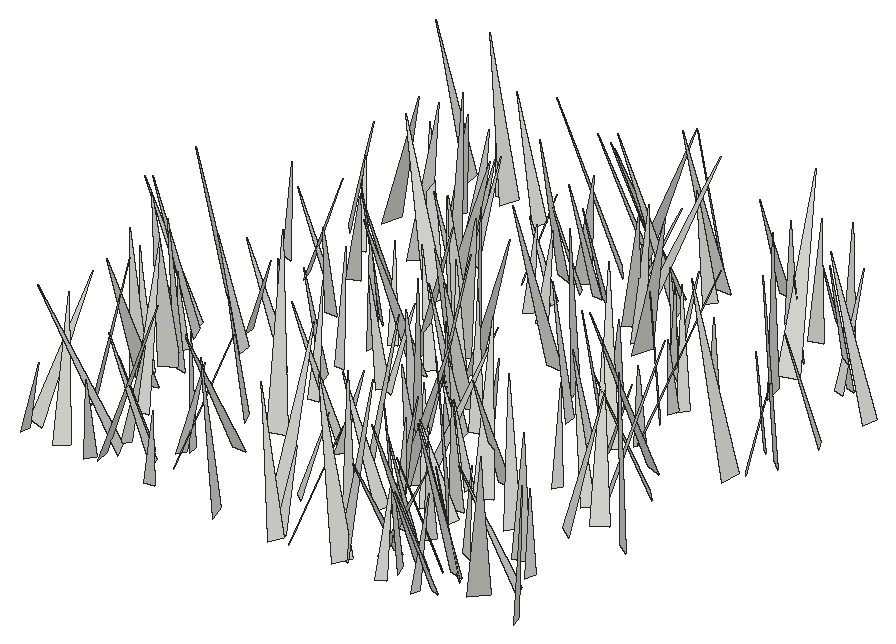
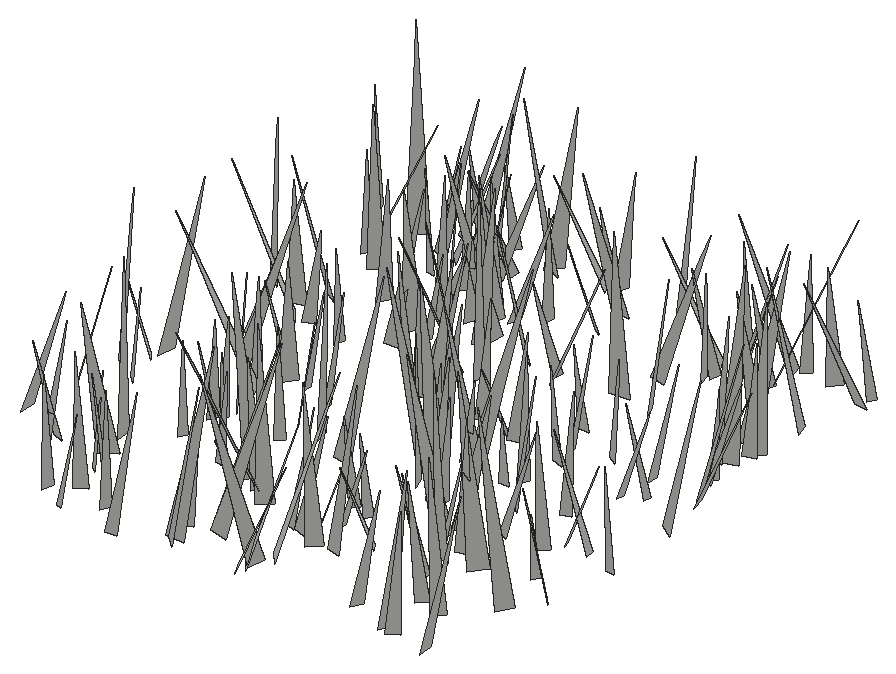
# SketchUp Ruby script. Lengths in inches.
U = 1.inch
M = Sketchup.active_model
def pt(a) = Geom::Point3d.new(a.map { |v| v * U })
def face(e, loops, mat)
  f = e.add_face(loops[0].map { |a| pt(a) })
  loops[1..].each { |l| e.add_face(l.map { |a| pt(a) }).erase! }
  f.material = f.back_material = mat if mat
  f
end
# faces: each face lists its corners as indices into pts; further lists are holes
def faces(e, pts, list, mat = nil) = list.each { |f| face(e, (f[0].is_a?(Array) ? f : [f]).map { |l| l.map { |i| pts[i] } }, mat) }
# xy, xz, yz: faces in a plane at the given z, y or x. An outline is a flat list of corners, or four numbers for a rectangle; further outlines are holes
def ring(l) = l.size == 4 ? [[l[0], l[1]], [l[2], l[1]], [l[2], l[3]], [l[0], l[3]]] : l.each_slice(2).to_a
def flat(e, list, mat, &to3) = list.each { |f| face(e, (f[0].is_a?(Array) ? f : [f]).map { |l| ring(l).map { |u, v| to3.(u, v) } }, mat) }
def xy(e, z, list, mat = nil) = flat(e, list, mat) { |x, y| [x, y, z] }
def xz(e, y, list, mat = nil) = flat(e, list, mat) { |x, z| [x, y, z] }
def yz(e, x, list, mat = nil) = flat(e, list, mat) { |y, z| [x, y, z] }
def lines(e, pts, list) = list.each { |a, b| e.add_line(pt(pts[a]), pt(pts[b])) }
# prism: a flat outline (further loops are holes) pulled along v
def prism(e, loops, v, mat = nil)
  f = face(e, loops, mat); d = Geom::Vector3d.new(v.map { |x| x * U })
  f.pushpull(f.normal.samedirection?(d) ? d.length : -d.length)
end
def box(e, o, s, mat = nil) = prism(e, [[o, [o[0] + s[0], o[1], o[2]], [o[0] + s[0], o[1] + s[1], o[2]], [o[0], o[1] + s[1], o[2]]]], [0, 0, s[2]], mat)
def at(x, y, z, deg = 0) = Geom::Transformation.translation(pt([x, y, z])) * Geom::Transformation.rotation(ORIGIN, Z_AXIS, deg.degrees)
def axes(o, x, y, z) = Geom::Transformation.new([*x, 0, *y, 0, *z, 0, *pt(o).to_a, 1])
def part(name) = M.definitions.add(name)
# library, detail: a bought-in or finely detailed component or shape, given as its bounding box
def library(name, o, s) = part(name).tap { |d| box(d.entities, o, s) }
def detail(e, o, s) = box(e.add_group.entities, o, s)
def put(e, d, t, mat = nil) = e.add_instance(d, t).tap { |i| i.material = mat if mat }
def group(e, t, mat = nil) = e.add_group.tap { |g| g.transformation = t; g.material = mat if mat }.entities
root = M.entities
c1 = part("fur_instance\#9")
p = [[0.8125,0,1.79],[0.67,-0.02,1.48],[0,-0.11,0],[0,0.11,0]]
faces(c1.entities,p,[[0,1,2,3]])
put(root,c1,axes([455.98,77.39,-21.66],[-6.00367,-1.40851,0.07652],[-1.40991,5.98159,-0.51624],[-0.04369,0.52005,6.14503]))
put(root,c1,axes([455.24,82.02,-21.66],[-3.32824,-5.52708,1.61735],[-5.74671,3.30884,-0.51825],[0.37393,1.65668,6.43096]))
put(root,c1,axes([454.55,89.52,-21.66],[-0.60793,-4.00143,1.69165],[-4.28266,0.83877,0.44495],[0.72934,1.58988,4.02282]))
put(root,c1,axes([456.5625,76.4,-21.66],[-6.28754,-2.52373,1.27093],[-2.51372,6.41179,0.29625],[1.29062,0.19325,6.76865]))
put(root,c1,axes([455.45,95.79,-21.66],[3.51843,3.11531,1.14482],[3.25687,-3.56198,-0.31656],[-0.63919,-1.00114,4.68874]))
put(root,c1,axes([457.41,74.3,-21.66],[-2.05359,-3.75931,0.63579],[-3.81243,2.01617,-0.39286],[-0.04503,0.74602,4.26559]))
put(root,c1,axes([455.75,58.35,-21.66],[1.29367,6.30142,0.29631],[6.29029,-1.26564,-0.54746],[0.47747,-0.39942,6.4095]))
put(root,c1,axes([457.89,107.22,-21.66],[-6.59248,-1.12335,1.64682],[-1.04061,6.79216,0.46743],[1.70031,-0.1986,6.67115]))
put(root,c1,axes([457.38,69.51,-21.66],[1.73924,-4.25815,2.51532],[-4.74882,-2.1825,-0.41111],[-1.38108,2.14207,4.58125]))
put(root,c1,axes([455.6875,57.11,-21.66],[3.70802,-0.97097,0.29213],[-0.94384,-3.70994,-0.3508],[-0.37053,-0.26665,3.81695]))
put(root,c1,axes([457.16,68.78,-21.66],[-4.56803,3.68378,2.77525],[4.20348,4.93276,0.37129],[1.89817,-2.05836,5.85656]))
put(root,c1,axes([457.33,73.82,-21.66],[2.92591,-1.89098,1.19539],[-1.88086,-3.14489,-0.37117],[-1.21125,0.31559,3.46396]))
put(root,c1,axes([458.28,93.65,-21.66],[-2.65941,2.49787,0.36396],[2.46932,2.68404,-0.37765],[0.52369,0.0288,3.62894]))
put(root,c1,axes([458.09,71.22,-21.66],[2.83404,-7.21043,2.36501],[-7.48804,-3.06648,-0.37599],[-1.22999,2.05469,7.73827]))
put(root,c1,axes([459.79,88.1,-21.66],[-3.92921,-1.09616,0.24918],[-1.11465,3.91653,-0.34741],[0.14562,0.40197,4.06442]))
put(root,c1,axes([456.86,63.92,-21.66],[6.14666,2.4589,1.36982],[2.59506,-6.2248,-0.47069],[-1.09008,-0.95377,6.60349]))
put(root,c1,axes([459,71.33,-21.66],[1.62899,5.48386,2.82302],[6.01922,-2.05055,0.50999],[-1.34582,-2.53344,5.69792]))
put(root,c1,axes([459.23,57.04,-21.66],[-4.06626,4.25963,1.22614],[4.27905,4.20638,-0.4224],[1.15655,-0.5867,5.87371]))
put(root,c1,axes([458.66,68.01,-21.66],[1.6119,-7.35068,0.1441],[-7.34568,-1.61634,-0.28263],[-0.30696,0.08011,7.52003]))
put(root,c1,axes([457.45,88.27,-21.66],[4.85217,1.44436,0.49792],[1.4914,-4.83766,-0.50049],[-0.33141,-0.62336,5.03778]))
put(root,c1,axes([457.14,98.72,-21.66],[7.07591,-3.11018,0.05148],[-3.09924,-7.06002,-0.5432],[-0.26559,-0.47663,7.71016]))
put(root,c1,axes([461.06,80.16,-21.66],[-4.01235,0.08097,0.58825],[0.14386,4.03101,0.42638],[0.5761,-0.44265,3.99045]))
put(root,c1,axes([460.87,76.62,-21.66],[-4.89796,-0.50596,1.28828],[-0.38248,5.0478,0.52832],[1.33018,-0.4116,4.8956]))
put(root,c1,axes([460.72,64.51,-21.66],[-0.70792,6.63222,0.94241],[6.69223,0.65809,0.39581],[-0.29764,-0.97786,6.65814]))
put(root,c1,axes([459.33,79.11,-21.66],[3.75751,0.05108,0.3502],[0.07903,-3.76142,-0.29936],[-0.34497,-0.30538,3.74592]))
put(root,c1,axes([463.09,59.12,-21.66],[-6.90561,-3.33755,0.10935],[-3.32242,6.89219,0.54573],[0.33571,-0.44394,7.65042]))
put(root,c1,axes([461.28,106.8125,-21.66],[2.88206,-3.90926,2.29022],[-4.22914,-3.29495,-0.30223],[-1.62535,1.64154,4.8474]))
put(root,c1,axes([462.29,106.21,-21.66],[-6.37075,2.32719,2.17346],[2.54476,6.64308,0.34616],[1.91413,-1.08621,6.77365]))
put(root,c1,axes([460.53,89.95,-21.66],[2.83156,-3.99697,0.33188],[-4.00855,-2.80696,0.39506],[0.13188,0.49882,4.88236]))
put(root,c1,axes([460.4,102.53,-21.66],[4.90607,-3.46037,0.24315],[-3.44997,-4.91123,-0.28332],[-0.36191,-0.09172,5.99695]))
put(root,c1,axes([462.11,56.84,-21.66],[3.06057,-3.28635,0.3748],[-3.27189,-3.08287,-0.31361],[-0.4851,0.05914,4.47983]))
put(root,c1,axes([462.46,84.85,-21.66],[0.91835,-4.65892,0.5996],[-4.68613,-0.86646,0.44487],[0.32448,0.67241,4.72768]))
put(root,c1,axes([464.28,90.08,-21.66],[-1.9055,-4.08481,0.78377],[-4.15591,1.83492,-0.5407],[-0.16841,0.93717,4.47485]))
put(root,c1,axes([462.74,60.28,-21.66],[4.01633,-1.15722,1.23996],[-1.33038,-4.12648,0.45808],[-1.05202,0.80037,4.15454]))
put(root,c1,axes([462.67,101.61,-21.66],[2.7967,-3.72992,1.22325],[-3.91864,-2.74089,0.60164],[-0.23004,1.34365,4.62297]))
put(root,c1,axes([462.46,95.28,-21.66],[5.72788,-5.11466,1.67521],[-5.30647,-5.77538,0.51083],[-0.89854,1.50329,7.66207]))
put(root,c1,axes([464.77,94.09,-21.66],[1.5886,-5.12639,3.23902],[-5.9044,-2.07062,-0.3813],[-1.38174,2.95423,5.35333]))
put(root,c1,axes([465.27,60.46,-21.66],[-3.54687,-2.63553,0.56126],[-2.61948,3.58991,0.30355],[0.63194,0.08835,4.40842]))
put(root,c1,axes([462.7,57.49,-21.66],[6.72772,1.76518,0.89994],[1.69777,-6.77807,0.60273],[-1.02144,0.36032,6.92927]))
put(root,c1,axes([465.0625,76.11,-21.66],[1.82668,3.73793,1.95155],[3.99067,-2.21946,0.51574],[-1.36206,-1.48974,4.1283]))
put(root,c1,axes([466.35,59.08,-21.66],[-5.39834,-1.72938,0.70035],[-1.70183,5.44274,0.32197],[0.76486,-0.09564,5.65943]))
put(root,c1,axes([466.17,105.02,-21.66],[-4.97411,1.9133,1.24146],[2.05101,5.05519,0.42681],[0.99764,-0.85328,5.31228]))
put(root,c1,axes([467.28,91.24,-21.66],[-6.20404,3.776,0.73856],[3.82283,6.20814,0.37243],[0.43544,-0.70326,7.25325]))
put(root,c1,axes([466.09,86.31,-21.66],[-3.7574,-4.18768,1.74578],[-4.4509,3.84178,-0.36412],[0.87968,1.55129,5.61445]))
put(root,c1,axes([464.91,98.61,-21.66],[3.97041,-1.42005,1.05601],[-1.57618,-4.01704,0.5243],[-0.80459,0.86179,4.18399]))
put(root,c1,axes([466.41,94.63,-21.66],[-3.79793,-0.43925,1.06155],[-0.29859,3.91782,0.55288],[1.10936,-0.44932,3.78306]))
put(root,c1,axes([465.59,95.71,-21.66],[-2.07525,-6.86081,3.30693],[-7.48887,2.46229,0.40886],[1.38687,3.02978,7.15613]))
put(root,c1,axes([466.04,97.37,-21.66],[1.29664,4.3065,0.97913],[4.41517,-1.23995,-0.39328],[0.1042,-1.05001,4.48024]))
put(root,c1,axes([467.3,62.46,-21.66],[-4.422,-0.95671,1.75223],[-1.16644,4.69405,-0.38074],[1.6202,0.76828,4.50826]))
put(root,c1,axes([467.46,68.69,-21.66],[-4.6895,-2.45579,1.69505],[-2.43913,4.97359,0.45768],[1.71894,0.35769,5.27378]))
put(root,c1,axes([467.99,79,-21.66],[0.81104,4.54834,1.26147],[4.65262,-0.98593,0.56355],[-0.7949,-1.13006,4.58559]))
put(root,c1,axes([468.2,77.04,-21.66],[-4.55771,-1.35516,1.4154],[-1.26006,4.77117,0.51063],[1.50069,-0.10962,4.72742]))
put(root,c1,axes([466.92,61.63,-21.66],[4.20297,-1.11156,0.80651],[-1.18233,-4.24977,0.30429],[-0.69867,0.5049,4.33681]))
put(root,c1,axes([469.01,84,-21.66],[-0.87591,3.86506,0.33078],[3.84564,0.82067,0.59405],[-0.50909,-0.4507,3.91829]))
put(root,c1,axes([468.09,82.85,-21.66],[4.81176,-1.3762,1.70282],[-1.26945,-5.10354,-0.53746],[-1.78382,-0.0803,4.97575]))
put(root,c1,axes([467.99,56.46,-21.66],[1.46502,-3.697,0.60293],[-3.73698,-1.39797,0.50827],[0.25762,0.74531,3.94408]))
put(root,c1,axes([469.58,73.9,-21.66],[-0.43977,4.5707,0.64422],[4.59918,0.3789,0.45132],[-0.39225,-0.6818,4.56957]))
put(root,c1,axes([469.91,64.72,-21.66],[-0.6438,-6.00502,0.1729],[-5.98541,0.62626,-0.53591],[-0.51472,0.22839,6.0156]))
put(root,c1,axes([467.79,59.82,-21.66],[5.23362,2.8594,0.35445],[2.818,-5.23298,0.60609],[-0.60055,0.36375,5.93293]))
put(root,c1,axes([467.59,93.05,-21.66],[6.355,-3.28716,0.66061],[-3.33311,-6.3472,0.48096],[-0.36352,0.73183,7.13864]))
put(root,c1,axes([470.67,68.27,-21.66],[-1.87564,7.62096,1.95831],[7.8685,1.80971,0.49369],[-0.027,-2.0194,7.83284]))
put(root,c1,axes([470.77,89.02,-21.66],[-4.87312,1.26006,1.29377],[1.19613,5.04128,-0.40455],[1.35309,0.08157,5.01711]))
put(root,c1,axes([470.54,97.42,-21.66],[3.10796,2.24348,0.34109],[2.21254,-3.12436,0.38987],[-0.50422,0.11876,3.81322]))
put(root,c1,axes([471.57,89.03,-21.66],[3.82096,-4.05561,2.24215],[-4.19487,-4.26194,-0.56033],[-1.96935,1.20949,5.5438]))
put(root,c1,axes([472.53,78.42,-21.66],[-2.40754,3.72637,1.88833],[4.14407,2.40561,0.53634],[0.52762,-1.89079,4.40391]))
put(root,c1,axes([473.53,82.77,-21.66],[-4.1604,2.35856,0.20079],[2.33408,4.15517,-0.44576],[0.39395,0.28953,4.76162]))
put(root,c1,axes([473.17,81.86,-21.66],[-0.92127,-7.60318,0.93237],[-7.64439,0.85236,-0.60268],[-0.49091,0.99576,7.63504]))
put(root,c1,axes([472.51,99.85,-21.66],[-2.15861,-6.19615,1.53511],[-6.31129,2.3146,0.46773],[0.95736,1.28794,6.5447]))
put(root,c1,axes([474.41,96.39,-21.66],[-3.5972,0.42819,0.55364],[0.48536,3.61469,0.35791],[0.50428,-0.42464,3.60487]))
put(root,c1,axes([473.23,78.2,-21.66],[1.4103,3.34023,0.25009],[3.32818,-1.428,0.30438],[-0.37801,-0.11091,3.61295]))
put(root,c1,axes([471.71,83.54,-21.66],[6.64605,0.23955,0.93352],[0.28653,-6.70181,-0.32012],[-0.92019,-0.35664,6.64266]))
put(root,c1,axes([476.02,69.38,-21.66],[-5.88175,-1.50758,0.15009],[-1.51502,5.85044,-0.60606],[-0.00586,0.62434,6.04156]))
put(root,c1,axes([475.32,103.32,-21.66],[-6.16047,-5.25921,0.96963],[-5.25018,6.22911,0.42963],[1.01736,0.29959,8.08864]))
put(root,c1,axes([474.88,98.91,-21.66],[-3.24657,-1.58505,0.39086],[-1.61743,3.24104,-0.29141],[0.22149,0.43432,3.60107]))
put(root,c1,axes([473.73,94.1875,-21.66],[-2.42915,2.39744,1.43013],[2.49267,2.71628,-0.31959],[1.25681,-0.75355,3.39799]))
put(root,c1,axes([474.66,56.12,-21.66],[-6.1633,-1.76581,2.36846],[-1.74431,6.59751,0.37966],[2.38433,0.26209,6.40002]))
put(root,c1,axes([474,87.9,-21.66],[5.47086,1.91538,2.35531],[2.21322,-5.83902,-0.39241],[-2.07794,-1.17628,5.78316]))
put(root,c1,axes([476.41,106.4375,-21.66],[-4.47388,-2.50611,0.21033],[-2.51468,4.46372,-0.30343],[0.03476,0.36756,5.119]))
put(root,c1,axes([474.44,84.8125,-21.66],[0.33482,-6.22736,0.74708],[-6.26175,-0.28913,0.39628],[0.3585,0.76592,6.22375]))
put(root,c1,axes([476.13,105.68,-21.66],[-4.87517,-3.87645,0.62854],[-3.83008,4.91477,0.6039],[0.86741,-0.08574,6.19915]))
put(root,c1,axes([475.68,83.64,-21.66],[-2.17723,3.86998,1.04919],[4.00343,2.16477,0.32287],[0.22393,-1.07466,4.42864]))
put(root,c1,axes([476.33,99.12,-21.66],[-1.41742,-4.71426,1.18858],[-4.85717,1.31918,-0.56008],[-0.21176,1.29675,4.89077]))
put(root,c1,axes([474.09,85.61,-21.66],[4.71855,-5.46855,1.25045],[-5.59838,-4.69426,0.59612],[-0.35606,1.33873,7.19821]))
put(root,c1,axes([474.16,100.02,-21.66],[4.15858,-4.6502,0.45845],[-4.67236,-4.14601,0.32855],[-0.05962,0.56087,6.22978]))
put(root,c1,axes([475.52,93.5,-21.66],[-1.6026,3.32948,1.45838],[3.48573,1.8596,-0.41502],[1.03054,-1.11225,3.67172]))
put(root,c1,axes([476.49,77.24,-21.66],[3.6689,-2.8215,1.45683],[-2.81207,-3.92099,-0.512],[-1.47496,0.45716,4.59995]))
put(root,c1,axes([476.11,68.76,-21.66],[3.72364,-1.08643,0.80362],[-1.21362,-3.72465,0.58799],[-0.59435,0.79892,3.83407]))
put(root,c1,axes([477.3,98.89,-21.66],[-1.94034,-4.30134,0.80925],[-4.30819,2.03312,0.47669],[0.77193,0.53502,4.69459]))
put(root,c1,axes([478.3125,58.63,-21.66],[0.44326,7.59594,0.73525],[7.62112,-0.4789,0.35297],[-0.39679,-0.71255,7.60067]))
put(root,c1,axes([475.81,104.82,-21.66],[7.43524,-1.67911,0.29476],[-1.69435,-7.42416,0.44731],[-0.18841,0.50147,7.60934]))
put(root,c1,axes([476.36,84.36,-21.66],[7.28234,-1.08518,0.65082],[-1.04869,-7.30325,-0.44316],[-0.70811,-0.34428,7.3494]))
put(root,c1,axes([477.91,61.79,-21.66],[2.28219,3.09258,0.57784],[3.14608,-2.24088,-0.43237],[0.01087,-0.72161,3.81909]))
put(root,c1,axes([480.58,55.74,-21.66],[-5.69821,2.17721,0.97614],[2.15034,5.78116,-0.34192],[1.034,-0.02439,6.0904]))
put(root,c1,axes([479.2,79.96,-21.66],[1.80262,-6.00522,1.15434],[-6.08405,-1.88243,-0.2921],[-0.61598,1.01901,6.26312]))
put(root,c1,axes([479.3125,68.36,-21.66],[3.26782,5.25044,1.3347],[5.28581,-3.43164,0.55786],[-1.18691,-0.82697,6.1591]))
put(root,c1,axes([478.1875,101.78,-21.66],[3.49532,2.40186,0.16337],[2.40303,-3.46356,-0.49202],[0.14512,-0.49771,4.21237]))
put(root,c1,axes([480.54,88.79,-21.66],[-1.04582,-7.4675,1.55674],[-7.62212,0.96116,-0.50998],[-0.30029,1.61039,7.52311]))
put(root,c1,axes([480.77,103.11,-21.66],[-1.44964,-7.72306,0.36058],[-7.72764,1.4358,-0.315],[-0.24346,0.41228,7.85162]))
put(root,c1,axes([478.87,76.05,-21.66],[-4.56158,-4.36485,4.54967],[-5.17144,5.80258,0.38189],[3.60662,2.79958,6.30192]))
put(root,c1,axes([482.51,101,-21.66],[-7.47727,-2.4998,1.10622],[-2.44373,7.5564,0.55783],[1.22512,-0.18436,7.86431]))
put(root,c1,axes([481.69,76.37,-21.66],[-6.39617,-0.72322,1.67284],[-0.5993,6.59982,0.56183],[1.72113,-0.38959,6.41236]))
put(root,c1,axes([480.3,56.59,-21.66],[1.50954,-3.07856,1.78204],[-3.55315,-1.39659,0.59714],[-0.16832,1.87187,3.37633]))
put(root,c1,axes([480.42,72.61,-21.66],[7.19679,1.10507,2.93039],[1.40985,-7.70082,-0.55845],[-2.79655,-1.03845,7.25969]))
put(root,c1,axes([480.7,75.97,-21.66],[-1.22041,-5.00142,1.71972],[-5.19067,1.47111,0.5948],[1.01418,1.51086,5.11369]))
put(root,c1,axes([481.83,62.8125,-21.66],[-5.13165,1.21269,1.54361],[1.09048,5.35359,-0.58061],[1.63224,0.23592,5.24093]))
put(root,c1,axes([482.12,77.52,-21.66],[-1.52023,5.3398,1.43684],[5.52962,1.4775,0.35965],[0.03531,-1.48075,5.54032]))
put(root,c1,axes([483.79,64.32,-21.66],[-5.48132,1.03762,0.48302],[1.07413,5.47965,0.41785],[0.39525,-0.50168,5.563]))
put(root,c1,axes([482.89,106.17,-21.66],[-4.49464,-4.79472,1.8462],[-5.03521,4.59856,-0.3156],[1.02201,1.56958,6.56442]))
put(root,c1,axes([482.9,105.59,-21.66],[-0.40917,-7.70862,1.45343],[-7.84037,0.35495,-0.32469],[-0.25296,1.46762,7.71264]))
put(root,c1,axes([481.02,97.3,-21.66],[3.73638,-5.69312,0.32255],[-5.69521,-3.70663,0.54933],[0.28337,0.57053,6.78752]))
put(root,c1,axes([482.87,95.76,-21.66],[4.88657,-1.90502,2.44295],[-2.30886,-5.28158,0.49977],[-2.06549,1.39696,5.22091]))
put(root,c1,axes([481.64,56.14,-21.66],[4.67763,2.46387,0.32375],[2.42875,-4.67875,0.51598],[-0.52599,0.30722,5.26162]))
put(root,c1,axes([483.39,103.625,-21.66],[3.00214,-3.52749,1.91618],[-3.65397,-3.39209,-0.51969],[-1.66236,1.08552,4.60282]))
put(root,c1,axes([484.96,72.53,-21.66],[-3.33504,1.53851,0.16438],[1.54705,3.32218,0.29368],[0.02564,-0.33558,3.66104]))
put(root,c1,axes([483.5,68.59,-21.66],[3.36896,-5.0045,1.18358],[-5.04079,-3.49374,-0.42432],[-1.01802,0.73793,6.01788]))
put(root,c1,axes([481.81,96.71,-21.66],[4.66085,6.54813,0.11631],[6.5407,-4.64683,-0.4912],[0.3329,-0.37945,8.02249]))
put(root,c1,axes([484.02,86.86,-21.66],[-6.46976,-1.55499,2.98827],[-1.52534,7.12153,0.40334],[3.00351,0.26714,6.64177]))
put(root,c1,axes([482.45,72.41,-21.66],[3.5807,5.01538,0.32607],[5.01642,-3.54168,-0.61141],[0.30977,-0.61982,6.13202]))
put(root,c1,axes([486.43,56.23,-21.66],[5.34271,-3.44394,4.19103],[-3.85612,-6.54857,-0.46545],[-3.8152,1.796,6.33945]))
put(root,c1,axes([486.3,66.42,-21.66],[-4.11869,2.39634,0.55767],[2.352,4.15398,-0.47915],[0.72219,0.13795,4.74094]))
put(root,c1,axes([486.34,83.34,-21.66],[-5.34365,-1.01248,1.41227],[-1.15776,5.47992,-0.452],[1.29585,0.72082,5.4199]))
put(root,c1,axes([483.18,67.4,-21.66],[7.44021,-1.05618,0.97458],[-1.13327,-7.472,0.55406],[-0.88376,0.68976,7.49435]))
put(root,c1,axes([484.74,75.53,-21.66],[4.77554,-0.30271,1.03368],[-0.19329,-4.86277,-0.53104],[-1.0596,-0.47722,4.75556]))
put(root,c1,axes([484.78,64.89,-21.66],[5.5976,-0.64404,1.05715],[-0.59203,-5.69245,-0.3332],[-1.08713,-0.21617,5.62467]))
put(root,c1,axes([486.54,86.45,-21.66],[-3.36264,-2.39418,1.21792],[-2.41208,3.55006,0.31902],[1.18208,0.43333,4.11555]))
put(root,c1,axes([484.07,94.74,-21.66],[7.12513,-3.29011,0.44393],[-3.26274,-7.13377,-0.50321],[-0.6135,-0.27186,7.83192]))
put(root,c1,axes([487.07,70.55,-21.66],[-3.6032,0.74818,1.09352],[0.87855,3.72087,0.34907],[0.99182,-0.57787,3.66346]))
put(root,c1,axes([486.12,56.78,-21.66],[3.51282,6.48869,2.15536],[6.79895,-3.57131,-0.32959],[-0.72316,-2.057,7.37118]))
put(root,c1,axes([487.35,94.6875,-21.66],[0.08392,3.77547,1.67654],[4.10941,-0.2474,0.35143],[-0.42151,-1.66031,3.76001]))
put(root,c1,axes([486.6,62.8125,-21.66],[0.02782,-4.7345,1.86898],[-5.06027,0.17616,0.52158],[0.54982,1.86087,4.70577]))
put(root,c1,axes([486.1875,89.03,-21.66],[1.68114,-3.92704,0.2758],[-3.91607,-1.63754,0.5539],[0.40264,0.46985,4.23569]))
put(root,c1,axes([487.04,108.01,-21.66],[-0.08674,-5.50292,0.32115],[-5.49794,0.10952,0.39174],[0.3974,0.31411,5.48965]))
put(root,c1,axes([489.18,65.98,-21.66],[-3.99444,1.28958,0.25526],[1.31279,3.95594,0.55757],[0.06915,-0.60932,4.16025]))
put(root,c1,axes([488.49,62.23,-21.66],[-4.19066,-2.50752,1.09961],[-2.47633,4.32875,0.43379],[1.16817,0.18082,4.86427]))
put(root,c1,axes([488.67,66.18,-21.66],[-5.61783,-2.93903,2.21928],[-3.25584,5.85535,-0.48739],[1.72124,1.48327,6.32142]))
put(root,c1,axes([488.71,70.08,-21.66],[-4.66477,5.25581,1.41142],[5.28211,4.8201,-0.49149],[1.30953,-0.72026,7.01013]))
put(root,c1,axes([488.82,59.9,-21.66],[-1.13114,-4.608,0.05517],[-4.59723,1.12439,-0.34274],[-0.31976,0.13515,4.73241]))
put(root,c1,axes([487.84,93.6875,-21.66],[-1.12295,-3.74744,1.45837],[-3.89173,1.39395,0.58526],[1.01223,1.20198,3.86805]))
put(root,c1,axes([488.2,67.57,-21.66],[1.13187,-5.42392,1.09616],[-5.52646,-1.05128,0.50466],[0.2806,1.17367,5.51773]))
put(root,c1,axes([488.7,72.8,-21.66],[-0.42981,-6.03201,0.26249],[-6.01913,0.44871,0.45551],[0.47339,0.22867,6.03012]))
put(root,c1,axes([489.37,81.8,-21.66],[-3.854,-0.48704,1.31581],[-0.33639,4.05498,0.51565],[1.36213,-0.37663,3.85028]))
put(root,c1,axes([488.26,93.35,-21.66],[2.5994,3.80823,1.24151],[3.99906,-2.55122,-0.54734],[-0.2268,-1.33772,4.57819]))
put(root,c1,axes([491.16,81.82,-21.66],[-5.19034,4.80556,0.45379],[4.78626,5.21014,-0.43029],[0.62529,0.00866,7.0603]))
put(root,c1,axes([490.65,57.875,-21.66],[-6.07164,-2.28107,2.04855],[-2.55827,6.27412,-0.5961],[1.68971,1.3026,6.45854]))
put(root,c1,axes([488.09,58.9375,-21.66],[4.49912,0.07902,0.02983],[0.07502,-4.46879,0.52292],[-0.03881,0.52233,4.46932]))
put(root,c1,axes([489.5,62.86,-21.66],[-3.20699,2.34244,2.63387],[2.95903,3.72406,0.29089],[1.91533,-1.83124,3.96071]))
put(root,c1,axes([489.75,105.22,-21.66],[4.11916,-1.93041,1.42636],[-1.9279,-4.34864,-0.31782],[-1.42975,0.30221,4.53795]))
put(root,c1,axes([490.47,55.8,-21.66],[-2.63101,2.88231,1.12737],[2.88894,2.81797,-0.46255],[1.11028,-0.50218,3.87505]))
put(root,c1,axes([491.45,59.4,-21.66],[-1.56855,-7.63886,0.47282],[-7.63369,1.59619,0.46371],[0.55001,0.36889,7.78444]))
put(root,c1,axes([492.02,89.66,-21.66],[-4.07522,2.66076,1.05763],[2.66001,4.19896,-0.31421],[1.05952,-0.30776,4.85678]))
put(root,c1,axes([491.48,87.54,-21.66],[-4.27511,-3.26782,2.05551],[-3.38668,4.64678,0.34365],[1.85313,0.95347,5.37002]))
put(root,c1,axes([492.99,59.83,-21.66],[-3.34237,-3.67886,0.49489],[-3.71061,3.29315,-0.58039],[-0.10119,0.75599,4.93646]))
put(root,c1,axes([491.87,74.89,-21.66],[3.56835,-1.26097,2.05366],[-1.59686,-3.9854,0.32755],[-1.80488,1.03305,3.77039]))
put(root,c1,axes([491.6,89.02,-21.66],[3.2467,-2.02133,0.75684],[-1.94033,-3.33216,-0.57574],[-0.94537,-0.10279,3.78092]))
put(root,c1,axes([493.25,67.91,-21.66],[-5.08391,3.17186,1.29588],[3.17676,5.23223,-0.34381],[1.28383,-0.38638,5.98237]))
put(root,c1,axes([492.17,93.08,-21.66],[3.31226,-1.52366,0.97308],[-1.49474,-3.45052,-0.31491],[-1.01694,0.10903,3.63228]))
put(root,c1,axes([492.66,107.16,-21.66],[-1.51621,-3.26203,0.55212],[-3.23761,1.58793,0.49084],[0.68086,0.28668,3.56354]))
put(root,c1,axes([491.64,81.11,-21.66],[3.71055,0.76796,0.33165],[0.80764,-3.68168,-0.51076],[-0.21789,-0.56867,3.7546]))
put(root,c1,axes([492.66,83.72,-21.66],[3.43508,-2.31671,0.74566],[-2.27877,-3.51457,-0.42176],[-0.85461,0.05948,4.12177]))
put(root,c1,axes([494.3,59.93,-21.66],[-2.38494,-6.16406,1.52656],[-6.35023,2.30898,-0.59758],[-0.0234,1.63919,6.58229]))
put(root,c1,axes([493.21,101.07,-21.66],[3.80415,1.70942,1.42934],[1.7089,-4.05302,0.29902],[-1.42996,-0.29602,4.15984]))
put(root,c1,axes([493.09,103.99,-21.66],[2.23095,-4.80055,1.901],[-5.14348,-2.24733,0.36107],[-0.45138,1.8816,5.28129]))
put(root,c1,axes([493.15,62.5625,-21.66],[-0.92871,-3.83483,1.6083],[-4.04735,1.2119,0.55253],[0.95473,1.40727,3.90681]))
put(root,c1,axes([494.71,56.875,-21.66],[-1.89303,-4.40404,0.51291],[-4.43222,1.86471,-0.34716],[-0.11875,0.60786,4.78107]))
put(root,c1,axes([493.5625,56,-21.66],[3.9323,-0.29865,1.47953],[-0.48436,-4.16008,0.44758],[-1.42954,0.58799,3.91814]))
put(root,c1,axes([494.91,59.46,-21.66],[-3.3946,-3.12525,1.18102],[-3.29173,3.41661,-0.4203],[0.5714,1.11577,4.59499]))
put(root,c1,axes([494.11,101.18,-21.66],[-2.25784,-3.06403,1.232],[-3.11024,2.47464,0.4545],[1.1102,0.70132,3.77883]))
put(root,c1,axes([494.85,98.55,-21.66],[-3.53884,7.24303,1.02774],[7.25201,3.62348,-0.56563],[0.96238,-0.67082,8.04145]))
put(root,c1,axes([495.49,74,-21.66],[-2.79772,3.91125,0.86225],[4.00509,2.73873,0.57209],[0.02536,-1.03446,4.77471]))
put(root,c1,axes([495.8,81.41,-21.66],[-3.1075,-6.9448,0.74353],[-6.98342,3.07514,-0.46373],[-0.12218,0.86773,7.5942]))
put(root,c1,axes([492.23,84.38,-21.66],[7.40183,3.33475,0.3809],[3.31775,-7.40888,0.39208],[-0.5081,0.20159,8.10888]))
put(root,c1,axes([495.06,105.4,-21.66],[4.42317,-1.03576,2.17466],[-1.28949,-4.85884,0.30856],[-2.03449,0.82776,4.53233]))
put(root,c1,axes([495.56,95.87,-21.66],[-6.42267,-1.42598,3.31634],[-1.29179,7.22813,0.60623],[3.37087,0.05298,6.55107]))
put(root,c1,axes([498,72.28,-21.66],[-2.69969,6.39263,0.77147],[6.43614,2.65406,0.5304],[-0.19237,-0.91623,6.91901]))
put(root,c1,axes([498.0625,78.23,-21.66],[-4.1053,-4.23157,0.31859],[-4.21802,4.11764,0.33835],[0.46467,-0.00766,5.88602]))
put(root,c1,axes([499.53,60.84,-21.66],[-5.35424,-1.86738,0.02315],[-1.86377,5.3475,0.29345],[0.11847,-0.26947,5.66294]))
put(root,c1,axes([496.68,64.57,-21.66],[2.3512,-5.85332,1.44977],[-6.03015,-2.28819,0.5412],[-0.02311,1.54732,6.28463]))
put(root,c1,axes([496.62,69.99,-21.66],[3.4607,5.10853,1.2476],[5.25066,-3.43918,-0.48234],[-0.29016,-1.30574,6.15149]))
put(root,c1,axes([496.96,73.86,-21.66],[5.77926,4.78065,0.80242],[4.74367,-5.8345,0.5954],[-0.99801,-0.04845,7.47663]))
put(root,c1,axes([499.65,99.91,-21.66],[-2.15143,-4.58063,1.63472],[-4.86135,2.07952,-0.57094],[0.14745,1.72526,5.02841]))
put(root,c1,axes([498.79,63.09,-21.66],[3.6892,-1.49713,1.29137],[-1.47127,-3.90506,-0.32413],[-1.32076,0.16824,3.96818]))
put(root,c1,axes([499.24,99.0625,-21.66],[1.25627,4.75609,0.70963],[4.78282,-1.31187,0.32531],[-0.49861,-0.60066,4.90844]))
put(root,c1,axes([501.01,83.95,-21.66],[-8.03417,0.61584,1.78735],[0.70083,8.21761,0.3188],[1.75577,-0.4621,8.05143]))
put(root,c1,axes([497.5625,58.47,-21.66],[5.80631,-5.6916,0.53269],[-5.68589,-5.82856,-0.29992],[-0.59055,0.15799,8.12513]))
put(root,c1,axes([500.46,88.77,-21.66],[-2.70575,-2.79772,1.42447],[-3.05403,2.78134,-0.3384],[0.7275,1.27058,3.87735]))
put(root,c1,axes([501.49,70.66,-21.66],[-3.98091,-5.38333,3.048],[-6.04161,4.16252,-0.53901],[1.33021,2.79489,6.67363]))
put(root,c1,axes([503.81,96.96,-21.66],[-6.67851,0.63047,0.27765],[0.60623,6.66388,-0.54986],[0.32721,0.52189,6.68563]))
put(root,c1,axes([502.37,87.68,-21.66],[-4.94486,-5.49387,2.91837],[-6.02867,5.15162,-0.51692],[1.53451,2.53562,7.37341]))
put(root,c1,axes([501.48,85.22,-21.66],[2.95559,2.2846,0.71516],[2.24296,-3.03986,0.44126],[-0.83663,-0.07885,3.70947]))
put(root,c1,axes([502.125,57.23,-21.66],[-4.83531,-1.63891,2.39644],[-2.01972,5.24312,-0.48946],[2.08559,1.27782,5.08199]))
put(root,c1,axes([503.12,91.96,-21.66],[-4.38014,-2.49103,0.91186],[-2.44951,4.47381,0.4553],[1.01814,0.04674,5.01832]))
